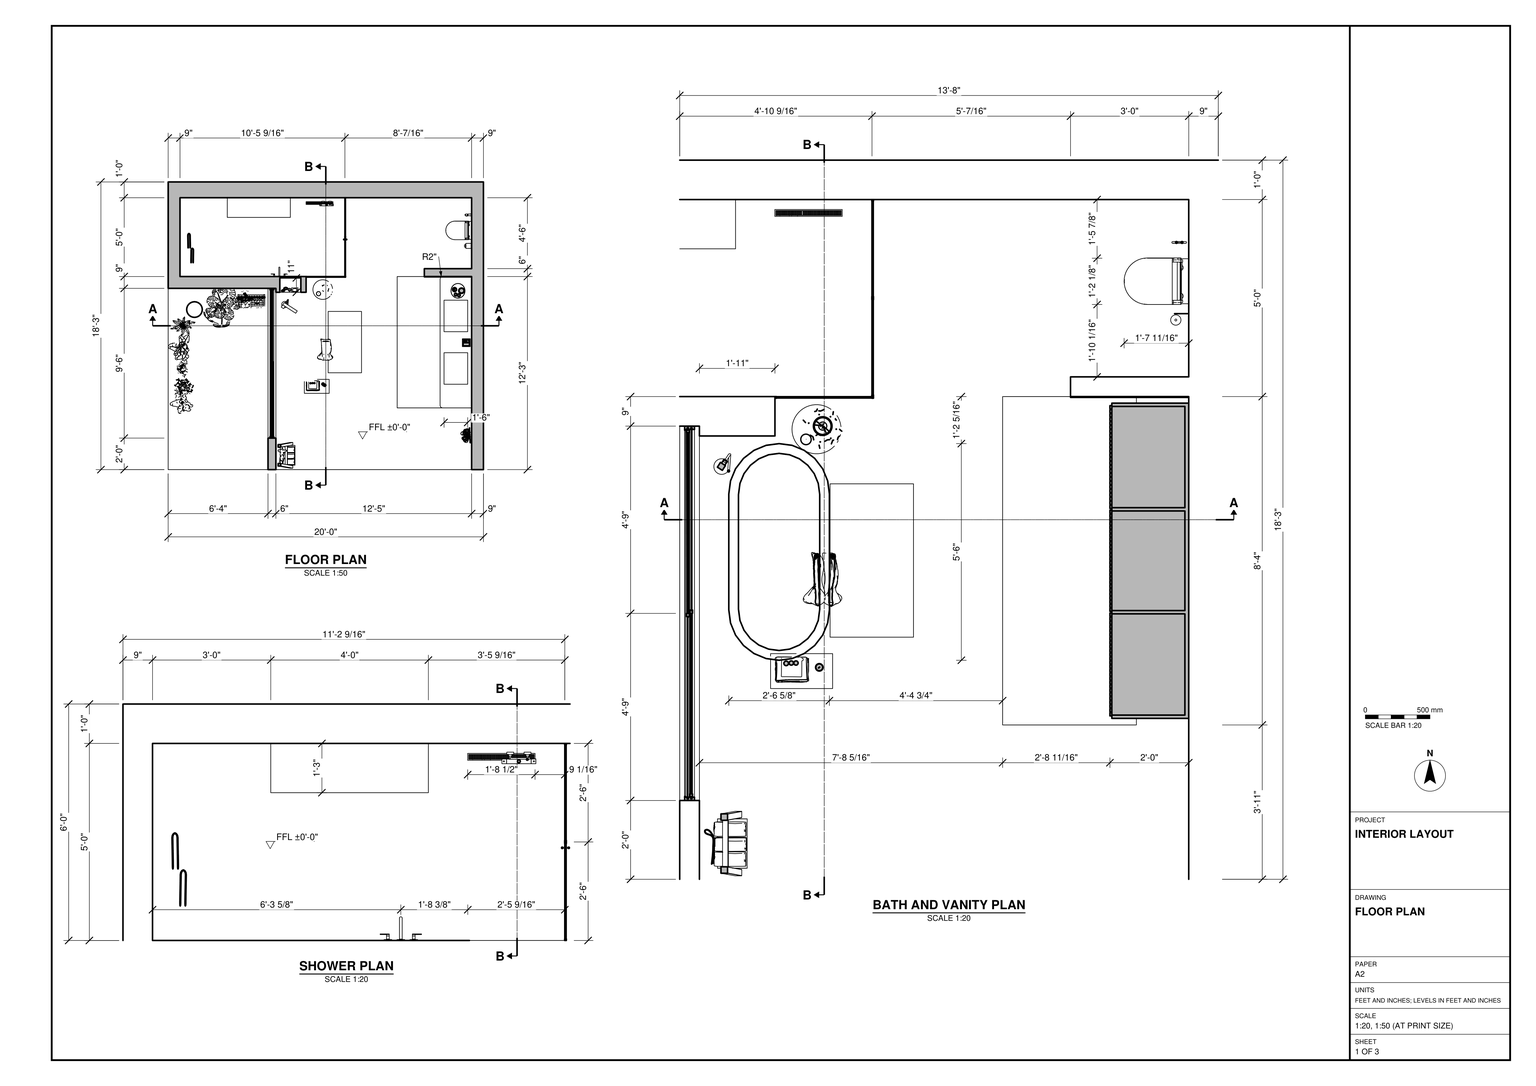
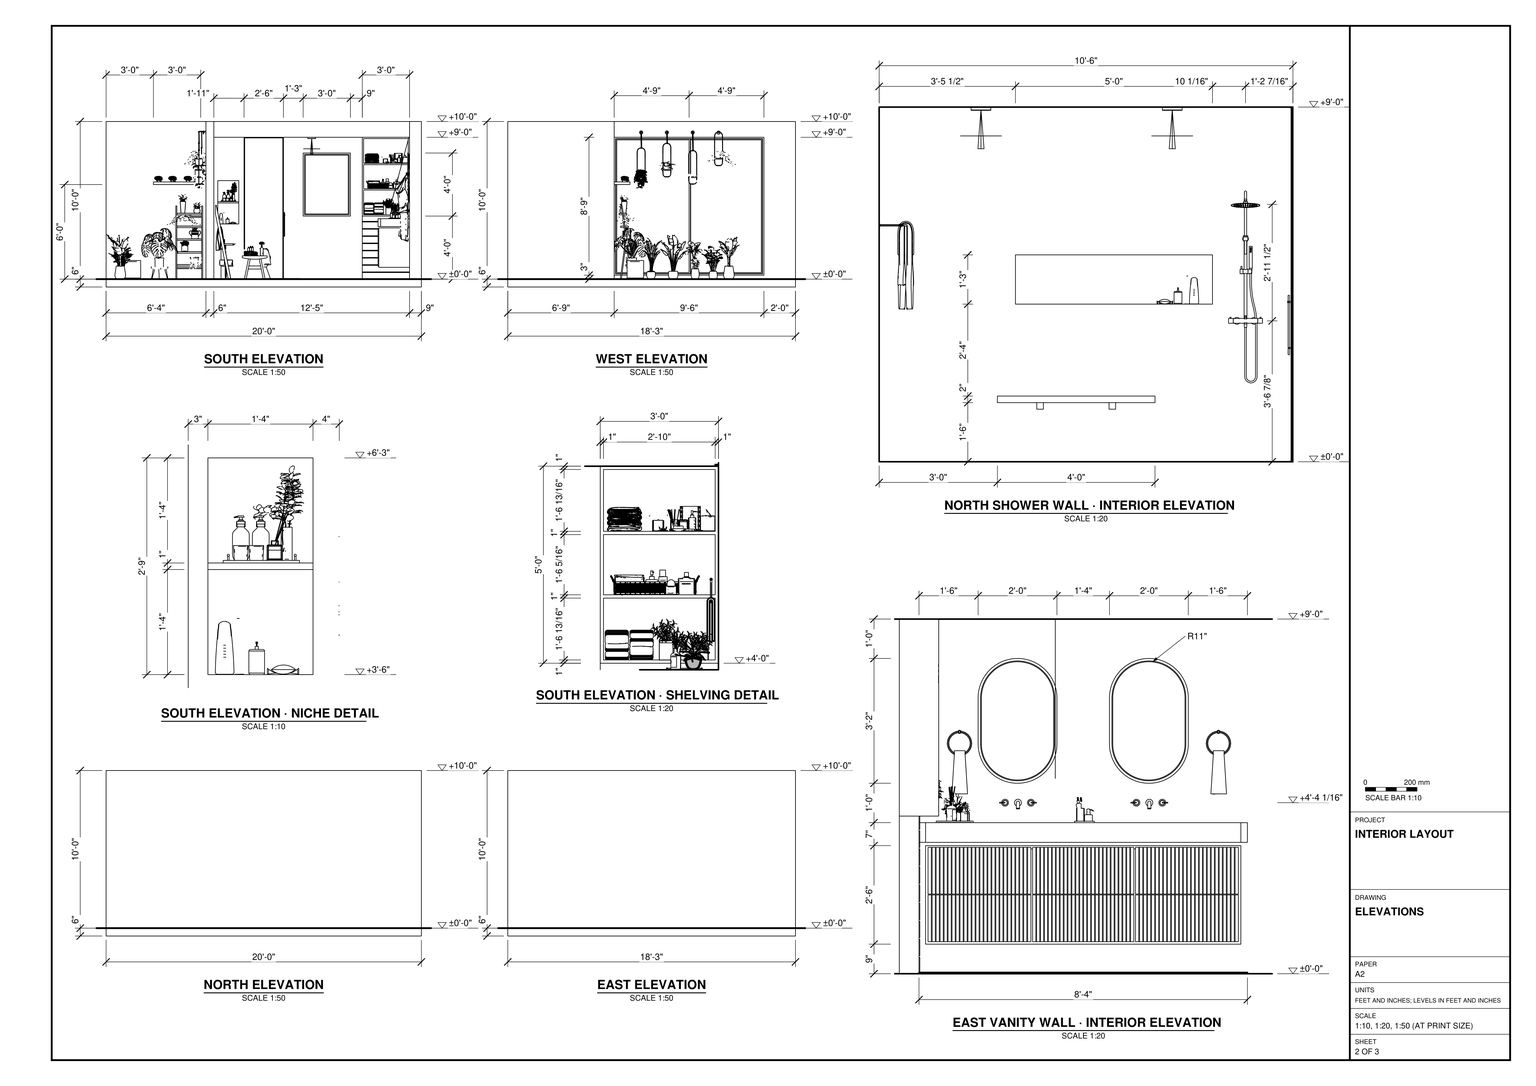
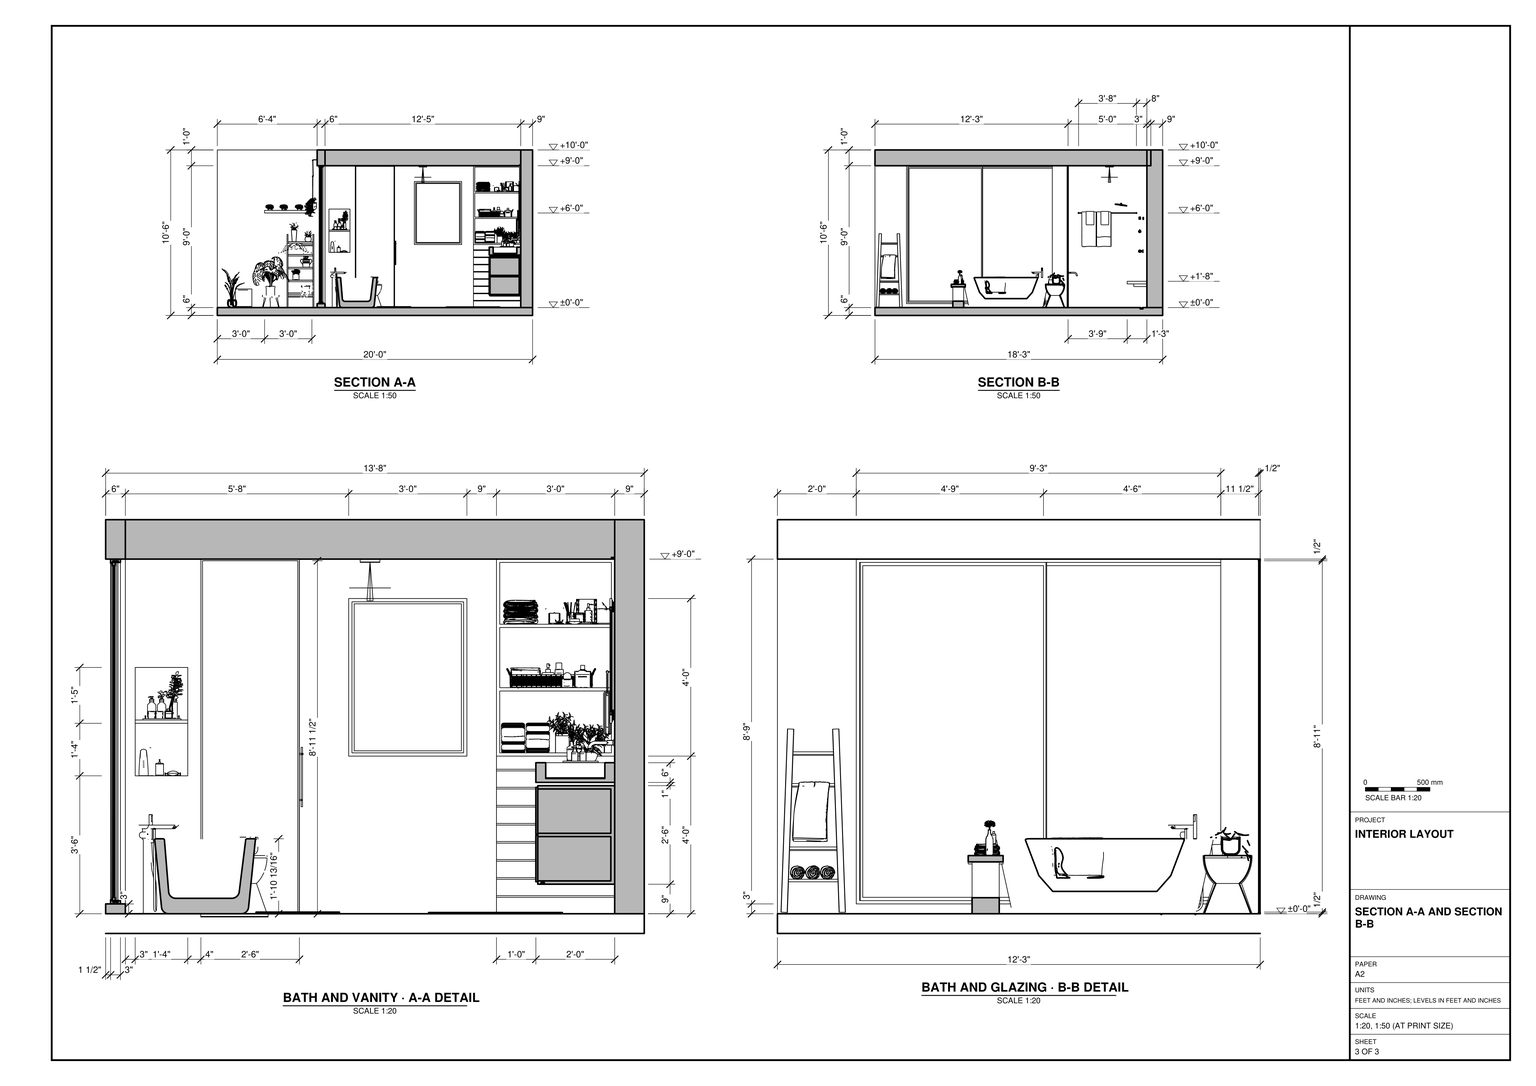
Build the bathroom interior in SketchUp from task_files/diagram_01.pdf. Work in feet and inches. The overall model is 20'-0" wide by 18'-3" deep by 10'-6" high, with the finished floor at ±0'-0". Use the floor plan to locate the walls, partitions and openings, and the sections to set their heights. Model the 6" floor slab and the 1'-0" overhead slab, keeping the planted area outside the enclosed bathroom as shown in section A-A.

Place the shower at the northwest corner and the toilet against the east wall in the northeast recess. Include the shower screen, fittings, wall recess and bench. Set the freestanding tub lengthwise beside the west glazing, facing the double vanity across the room. Use the enlarged plans and elevations to size the tub, the raised vanity cabinet, its countertop and basins, and the mirrors above. Detail the open shelving and the divided wall niche as shown in section A-A. Include the towel stand, bath-side accessories and planting where shown.

Decor and loose items may be any suitable library components. Keep the walls, slabs, roof and each furniture or joinery piece in separate groups or components, and use components for repeated parts. Save one SketchUp model as output_files/bathroom_with_a_freestanding_tub_and_double_vanity.skp.

# SketchUp Ruby script. Lengths in inches.
U = 1.inch
M = Sketchup.active_model
def pt(a) = Geom::Point3d.new(a.map { |v| v * U })
def face(e, loops, mat)
  f = e.add_face(loops[0].map { |a| pt(a) })
  loops[1..].each { |l| e.add_face(l.map { |a| pt(a) }).erase! }
  f.material = f.back_material = mat if mat
  f
end
# faces: each face lists its corners as indices into pts; further lists are holes
def faces(e, pts, list, mat = nil) = list.each { |f| face(e, (f[0].is_a?(Array) ? f : [f]).map { |l| l.map { |i| pts[i] } }, mat) }
# xy, xz, yz: faces in a plane at the given z, y or x. An outline is a flat list of corners, or four numbers for a rectangle; further outlines are holes
def ring(l) = l.size == 4 ? [[l[0], l[1]], [l[2], l[1]], [l[2], l[3]], [l[0], l[3]]] : l.each_slice(2).to_a
def flat(e, list, mat, &to3) = list.each { |f| face(e, (f[0].is_a?(Array) ? f : [f]).map { |l| ring(l).map { |u, v| to3.(u, v) } }, mat) }
def xy(e, z, list, mat = nil) = flat(e, list, mat) { |x, y| [x, y, z] }
def xz(e, y, list, mat = nil) = flat(e, list, mat) { |x, z| [x, y, z] }
def yz(e, x, list, mat = nil) = flat(e, list, mat) { |y, z| [x, y, z] }
def lines(e, pts, list) = list.each { |a, b| e.add_line(pt(pts[a]), pt(pts[b])) }
# prism: a flat outline (further loops are holes) pulled along v
def prism(e, loops, v, mat = nil)
  f = face(e, loops, mat); d = Geom::Vector3d.new(v.map { |x| x * U })
  f.pushpull(f.normal.samedirection?(d) ? d.length : -d.length)
end
def box(e, o, s, mat = nil) = prism(e, [[o, [o[0] + s[0], o[1], o[2]], [o[0] + s[0], o[1] + s[1], o[2]], [o[0], o[1] + s[1], o[2]]]], [0, 0, s[2]], mat)
def at(x, y, z, deg = 0) = Geom::Transformation.translation(pt([x, y, z])) * Geom::Transformation.rotation(ORIGIN, Z_AXIS, deg.degrees)
def axes(o, x, y, z) = Geom::Transformation.new([*x, 0, *y, 0, *z, 0, *pt(o).to_a, 1])
def part(name) = M.definitions.add(name)
# library, detail: a bought-in or finely detailed component or shape, given as its bounding box
def library(name, o, s) = part(name).tap { |d| box(d.entities, o, s) }
def detail(e, o, s) = box(e.add_group.entities, o, s)
def put(e, d, t, mat = nil) = e.add_instance(d, t).tap { |i| i.material = mat if mat }
def group(e, t, mat = nil) = e.add_group.tap { |g| g.transformation = t; g.material = mat if mat }.entities
root = M.entities
M.materials.add("1467 AP 9475 Shining Blue").color = [208, 218, 214]
M.materials.add("BANANA_BIG_STVOL_1").color = [93, 83, 53]
M.materials.add("Goldfish-custom-shape__54193.1487305638").color = [111, 138, 137]
M.materials.add("POT_TEXTURE_1").color = [172, 172, 172]
M.materials.add("POT_TEXTURE_2").color = [160, 154, 144]
M.materials.add("Shelves Light").color = [249, 232, 196]
M.materials.add("Steel_ Copper_ Metal_ Aluminium").color = [30, 30, 30]
M.materials.add("[Carrera Marble]").color = [207, 207, 207]
M.materials.add("[Color A01]").color = [127, 123, 119]
M.materials.add("[Marble Carrara Gold Floor Tile]").color = [221, 221, 221]
M.materials.add("[Metal Seamed]").color = [67, 65, 65]
M.materials.add("[Stone Brushed Khaki]").color = [196, 204, 211]
M.materials.add("[Tile Travertine 2 inch]").color = [56, 54, 50]
M.materials.add("[Wood Floor]").color = [107, 58, 35]
M.materials.add("[Wood Veneer 01]").color = [87, 43, 40]
M.materials.add("[Wood Veneer 01]1").color = [120, 70, 37]
M.materials.add("soil1").color = [68, 55, 47]
M.materials.add("white_concrete_pot1").color = [212, 211, 204]
M.materials.add("wood_1").color = [140, 119, 94]
c1 = library("skp31A6",[-6.04,-1.48,32.125],[7.16,7.43,5.2])
c2 = library("t3",[21.64,8.43,0],[7.57,4.96,6.27])
c3 = library("bathroom accessories",[-9.65,-7.51,0],[20.13,16.97,7.61])
c4 = library("interior plants_leaves_small",[-1.83,-3.05,0],[40.47,20.87,24.79])
c5 = library("Wall hung toilet",[0.42,0,0],[26.94,19.69,42.125])
c6 = library("bain4",[0,0,0],[65.98,62.12,30.23])
c7 = library("Bathroom stool",[0,0,0],[19.9375,11.76,29.04])
c8 = library("JEE-O slimline shower set bronze\#1",[0.04,-0.03,-18.98],[11.61,24.11,65.69])
c9 = part("Goldfish Aqua Runner")
box(c9.entities,[0,0,0],[43.79,100,0.375],"Goldfish-custom-shape__54193.1487305638")
c10 = library("Wall Tap 1",[0,0,0],[12.6,7.22,3.6875])
c11 = library("Hand Towel on Rack",[0,0,0],[3.03,7.5,19.47])
c12 = library("Untitled",[118.83,25.61,-0.38],[19.68,14.54,56.29])
c13 = library("Bathrobe with hooks",[0,0,-0.08],[18.125,10.02,52.34])
c14 = library("Perspective CM",[-13.58,-5.03,0],[27.16,11.23,7.55])
c15 = library("Bathroom accessories \#1",[0,0,0],[11.95,10.24,10.01])
c16 = library("Bahtoorm accessories \#2",[0,1.49,0],[12.27,10,14.78])
c17 = library("Untitled\#1",[35.54,-0.34,0],[6.02,6,7.73])
c18 = library("Bathroom Stool and Styling",[15.82,12.47,0],[25.92,25.93,28.18])
c19 = library("Scara cu plante",[-7.66,-9.41,-0.15],[30.59,22.83,66.38])
c20 = library("plant\#1",[-21.34,-27.21,-0.38],[41.91,41.15,38.97])
c21 = library("Plant\#2",[0,0,0],[12.59,12.59,14.16])
c22 = library("Group\#119",[-312.76,2118.02,370.79],[80.37,61.43,57.53])
c23 = library("Group\#164",[-146.29,2044.53,349.125],[81,53.32,37.9])
c24 = library("Group\#231",[-236.03,2064.57,238.29],[378.97,266.89,1422.96])
c25 = library("Group\#132",[-392.38,2142.99,345.23],[79.77,60.6,39.05])
c26 = library("Group\#193",[-390.04,2074.71,363.78],[77.3,84.83,61.55])
c27 = library("Group\#142",[-389.63,2051.04,359.41],[56.81,81.38,37.86])
c28 = library("Group\#146",[-362.86,1963.26,351.01],[55.56,80.44,37.9])
c29 = library("Group\#163",[-200.52,1998.86,370.22],[77.15,68.38,35.39])
c30 = library("Group\#184",[-480.58,1843.32,11.96],[467.85,466.24,378.92])
c31 = library("Group\#133",[-433.57,2042.61,369.7],[71.79,72.8,37.85])
c32 = library("Group\#130",[-148.5,2084.1,354.63],[73.89,71.73,39.48])
c33 = library("Group\#205",[-372.4375,2154.5,374],[76.125,67.08,39.0625])
c34 = library("Group\#206",[-275.5,2156.34,352.11],[71.39,73.27,44.69])
c35 = library("Group\#174",[-143.56,2061.14,371.42],[79.79,63.19,51.3])
c36 = library("Group\#192",[-363.89,1895.22,354.63],[76.92,66.54,39.48])
c37 = library("Group\#176",[-145.08,2015.32,369.99],[82.29,54.05,37.9])
c38 = library("Group\#203",[-315.77,2202.04,371],[80.74,54.44,37.85])
c39 = library("Group\#194",[-419.21,1941.11,355.02],[73.1,71.21,39.06])
c40 = library("Group\#199",[-229.79,1894.04,351.01],[79.82,63.55,37.9])
c41 = library("Group\#210",[-234.26,2180.97,367.05],[50.63,74.65,43.95])
c42 = library("Group\#213",[-904.81,1865.01,156.3],[624.43,217.34,1227.7])
c43 = library("Group\#214",[-312.51,1611.52,263.78],[120.52,408.52,1275.1])
c44 = library("Group\#217",[-571.16,1736.08,232.33],[294.08,306.57,1438.75])
c45 = library("Group\#222",[-273.21,1593.22,47.51],[374.54,419.07,1416.6])
c46 = library("Group\#123",[-202.35,1900.5,372.29],[58.53,80.11,50.06])
c47 = library("Group\#135",[-432.01,1984.38,372.6875],[64.1,75.95,39.0625])
c48 = library("Group\#168",[-310.7,1952.62,354.63],[79.53,58.52,39.48])
c49 = library("Group\#134",[-374.28,1979.7,369.99],[51.81,82.66,37.9])
c50 = library("Group\#201",[-397.18,1916.74,372.44],[70.02,74.57,49.25])
c51 = library("Group\#208",[-236.3,2186.8,344.47],[79.26,62.91,39.06])
c52 = library("Group\#122",[-161.07,2117.49,373.61],[81.25,53.73,39.48])
c53 = library("Group\#212",[-431.9,1883.46,368.72],[373.65,376.39,18.61])
c54 = library("Group\#167",[-340.96,1970.4,361.28],[81.22,51.59,61.62])
c55 = library("Group\#179",[-272.7,1884.51,369.99],[80.39,55.87,37.9])
c56 = library("Group\#153",[-330.83,2117.69,370.2],[61.83,80.2,35.55])
c57 = library("Group\#209",[-366.3125,2177.8,359.41],[79.9,61.23,37.86])
c58 = library("Group\#145",[-435.875,2067.96,347.82],[58.32,80.53,38.29])
c59 = library("Group\#207",[-183.79,2161.45,371.25],[72.43,70.21,54.35])
c60 = library("Group\#221",[-208.23,2037.18,75.37],[621.09,225.61,1251.82])
c61 = library("Group\#225",[-675.58,1862.05,152.55],[378.81,196.01,1743.84])
c62 = library("Group\#226",[-257.06,2048.08,160.05],[394.6,177.93,1743.83])
c63 = library("Group\#228",[-344.84,1500.61,160.55],[176.35,551.19,1921.45])
c64 = library("Group\#229",[-231.77,1913.24,119.96],[448.93,143.84,1582.05])
c65 = library("Group\#230",[-616.67,2098.6,178.29],[331.19,111.16,1177.92])
c66 = library("Group\#223",[-527.15,2088.47,150.96],[267.01,328.12,1599.25])
c67 = library("Group\#232",[-792.12,2067.32,152.13],[549.56,259.52,1931.8])
c68 = library("Group\#234",[-281.17,2118.67,243.77],[133.23,408.71,1313.3])
c69 = part("Potted houseplant \#1")
g1 = group(c69.entities,at(904.81,-1500.61,-11.96),"white_concrete_pot1")
detail(g1,[-222.14,2117.95,372.07],[61.87,75.41,50.35])
put(c69.entities,c22,at(904.81,-1500.61,-11.96),"white_concrete_pot1")
g2 = group(c69.entities,at(904.81,-1500.61,-11.96),"white_concrete_pot1")
detail(g2,[-313.93,1881.02,351.21],[70.15,73.18,37.2])
g3 = group(c69.entities,at(904.81,-1500.61,-11.96),"white_concrete_pot1")
detail(g3,[-209.1,1970.26,378.89],[50.57,81.04,37.2])
put(c69.entities,c23,at(904.81,-1500.61,-11.96),"white_concrete_pot1")
put(c69.entities,c24,at(904.81,-1500.61,-11.96))
put(c69.entities,c25,at(904.81,-1500.61,-11.96),"white_concrete_pot1")
put(c69.entities,c26,at(904.81,-1500.61,-11.96),"white_concrete_pot1")
put(c69.entities,c27,at(904.81,-1500.61,-11.96),"white_concrete_pot1")
put(c69.entities,c28,at(904.81,-1500.61,-11.96),"white_concrete_pot1")
g4 = group(c69.entities,at(904.81,-1500.61,-11.96),"white_concrete_pot1")
detail(g4,[-129.49,1972.75,359.91],[55.59,80.76,37.2])
put(c69.entities,c29,at(904.81,-1500.61,-11.96),"white_concrete_pot1")
g5 = group(c69.entities,at(904.81,-1500.61,-11.96),"white_concrete_pot1")
detail(g5,[-333.13,1892.25,370.19],[61.39,79.4,37.2])
put(c69.entities,c30,at(904.81,-1500.61,-11.96),"POT_TEXTURE_1")
put(c69.entities,c31,at(904.81,-1500.61,-11.96),"white_concrete_pot1")
put(c69.entities,c32,at(904.81,-1500.61,-11.96),"white_concrete_pot1")
g6 = group(c69.entities,at(904.81,-1500.61,-11.96),"white_concrete_pot1")
detail(g6,[-270.91,2176.57,345.18],[52.11,82.01,38.29])
g7 = group(c69.entities,at(904.81,-1500.61,-11.96),"white_concrete_pot1")
detail(g7,[-195.71,2019.1875,371.11],[58.98,81.18,37.2])
g8 = group(c69.entities,at(904.81,-1500.61,-11.96),"white_concrete_pot1")
detail(g8,[-319.36,2078.81,339.18],[76.07,69.08,39.48])
put(c69.entities,c33,at(904.81,-1500.61,-11.96),"white_concrete_pot1")
put(c69.entities,c34,at(904.81,-1500.61,-11.96),"white_concrete_pot1")
g9 = group(c69.entities,at(904.81,-1500.61,-11.96),"white_concrete_pot1")
detail(g9,[-417.64,2112.53,369.82],[65.44,79.59,38.29])
put(c69.entities,c35,at(904.81,-1500.61,-11.96),"white_concrete_pot1")
put(c69.entities,c36,at(904.81,-1500.61,-11.96),"white_concrete_pot1")
put(c69.entities,c37,at(904.81,-1500.61,-11.96),"white_concrete_pot1")
g10 = group(c69.entities,at(904.81,-1500.61,-11.96),"white_concrete_pot1")
detail(g10,[-240.6,2054.85,378.89],[71.5,72.03,37.2])
put(c69.entities,c38,at(904.81,-1500.61,-11.96),"white_concrete_pot1")
put(c69.entities,c39,at(904.81,-1500.61,-11.96),"white_concrete_pot1")
put(c69.entities,c40,at(904.81,-1500.61,-11.96),"white_concrete_pot1")
g11 = group(c69.entities,at(904.81,-1500.61,-11.96),"white_concrete_pot1")
detail(g11,[-249.82,2117.53,359.91],[58.07,81.25,37.2])
put(c69.entities,c41,at(904.81,-1500.61,-11.96),"white_concrete_pot1")
put(c69.entities,c42,at(904.81,-1500.61,-11.96))
put(c69.entities,c43,at(904.81,-1500.61,-11.96))
put(c69.entities,c44,at(904.81,-1500.61,-11.96))
put(c69.entities,c45,at(904.81,-1500.61,-11.96))
g12 = group(c69.entities,at(904.81,-1500.61,-11.96),"white_concrete_pot1")
detail(g12,[-435.4375,2027.54,350.71],[78.74,62.6,37.86])
put(c69.entities,c46,at(904.81,-1500.61,-11.96),"white_concrete_pot1")
g13 = group(c69.entities,at(904.81,-1500.61,-11.96),"white_concrete_pot1")
detail(g13,[-173.8,2126.25,354.63],[80.17,60.53,39.48])
g14 = group(c69.entities,at(904.81,-1500.61,-11.96),"white_concrete_pot1")
detail(g14,[-222.96,2066.75,359.91],[63.77,78.21,37.2])
put(c69.entities,c47,at(904.81,-1500.61,-11.96),"white_concrete_pot1")
g15 = group(c69.entities,at(904.81,-1500.61,-11.96),"white_concrete_pot1")
detail(g15,[-183.125,1913.38,330.04],[66.78,77.69,39.48])
put(c69.entities,c48,at(904.81,-1500.61,-11.96),"white_concrete_pot1")
g16 = group(c69.entities,at(904.81,-1500.61,-11.96),"white_concrete_pot1")
detail(g16,[-152,1936.85,378.89],[64.46,79.76,37.2])
g17 = group(c69.entities,at(904.81,-1500.61,-11.96),"white_concrete_pot1")
detail(g17,[-284.65,1933.22,373.64],[80.83,55.23,37.2])
put(c69.entities,c49,at(904.81,-1500.61,-11.96),"white_concrete_pot1")
g18 = group(c69.entities,at(904.81,-1500.61,-11.96),"white_concrete_pot1")
detail(g18,[-263.49,1923.54,359.91],[75.98,66.75,37.2])
put(c69.entities,c50,at(904.81,-1500.61,-11.96),"white_concrete_pot1")
g19 = group(c69.entities,at(904.81,-1500.61,-11.96),"white_concrete_pot1")
detail(g19,[-167.97,1940.97,354.63],[66.78,77.7,39.48])
put(c69.entities,c51,at(904.81,-1500.61,-11.96),"white_concrete_pot1")
g20 = group(c69.entities,at(904.81,-1500.61,-11.96),"white_concrete_pot1")
detail(g20,[-214.75,1956.59,330.04],[66.78,77.69,39.48])
put(c69.entities,c52,at(904.81,-1500.61,-11.96),"white_concrete_pot1")
put(c69.entities,c53,at(904.81,-1500.61,-11.96),"white_concrete_pot1")
put(c69.entities,c54,at(904.81,-1500.61,-11.96),"white_concrete_pot1")
g21 = group(c69.entities,at(904.81,-1500.61,-11.96),"white_concrete_pot1")
detail(g21,[-282.5625,1934.21,389.56],[81.1,59.19,35.03])
put(c69.entities,c55,at(904.81,-1500.61,-11.96),"white_concrete_pot1")
g22 = group(c69.entities,at(904.81,-1500.61,-11.96),"white_concrete_pot1")
detail(g22,[-394.5,2036.48,359.91],[79.58,64.84,37.2])
put(c69.entities,c56,at(904.81,-1500.61,-11.96),"white_concrete_pot1")
put(c69.entities,c57,at(904.81,-1500.61,-11.96),"white_concrete_pot1")
put(c69.entities,c58,at(904.81,-1500.61,-11.96),"white_concrete_pot1")
put(c69.entities,c59,at(904.81,-1500.61,-11.96),"white_concrete_pot1")
put(c69.entities,c60,at(904.81,-1500.61,-11.96))
put(c69.entities,c61,at(904.81,-1500.61,-11.96))
put(c69.entities,c62,at(904.81,-1500.61,-11.96))
put(c69.entities,c63,at(904.81,-1500.61,-11.96))
put(c69.entities,c64,at(904.81,-1500.61,-11.96))
put(c69.entities,c65,at(904.81,-1500.61,-11.96))
put(c69.entities,c66,at(904.81,-1500.61,-11.96))
put(c69.entities,c67,at(904.81,-1500.61,-11.96))
put(c69.entities,c68,at(904.81,-1500.61,-11.96))
c70 = library("Group\#242",[-662.41,217.3,320.04],[397.32,658.3,1732.06])
c71 = library("Group\#244",[-299.2,181.55,262.58],[360.65,735.71,1258.34])
c72 = library("Group\#239",[-1038.76,656.55,345.34],[733.18,460.51,2065.7])
c73 = library("Group\#237",[-445.29,890.31,329.28],[284.3,304.08,2023.29])
c74 = library("Group\#240",[-733.48,439.625,202.64],[456.28,533.12,1536.78])
c75 = library("Group\#243",[-455.56,899.32,410.78],[341.21,610.33,1581.5])
c76 = library("Group\#236",[-516.34,626.77,-4.5625],[517.73,515.95,418.98])
c77 = library("Group\#241",[-249.24,914.85,310.18],[345.55,647.95,1307.93])
c78 = library("Group\#238",[-277.97,488.68,287.26],[362.84,405.94,1768.54])
c79 = library("Group\#235",[-468.76,669.89,380.1875],[424.36,427.47,41.99])
c80 = part("Potted tropical plant")
put(c80.entities,c70,at(1038.76,-181.55,4.5625))
put(c80.entities,c71,at(1038.76,-181.55,4.5625))
put(c80.entities,c72,at(1038.76,-181.55,4.5625))
put(c80.entities,c73,at(1038.76,-181.55,4.5625))
put(c80.entities,c74,at(1038.76,-181.55,4.5625))
put(c80.entities,c75,at(1038.76,-181.55,4.5625))
put(c80.entities,c76,at(1038.76,-181.55,4.5625),"POT_TEXTURE_1")
put(c80.entities,c77,at(1038.76,-181.55,4.5625))
put(c80.entities,c78,at(1038.76,-181.55,4.5625))
put(c80.entities,c79,at(1038.76,-181.55,4.5625),"soil1")
c81 = library("Group\#248",[-246.45,-349.05,558.47],[136.91,100.49,66.1])
c82 = library("Group\#251",[-264.68,-415.73,1484.11],[304.64,209.69,227.41])
c83 = library("Group\#259",[-357.04,-394.18,1447.05],[213.62,306.36,356.95])
c84 = library("Group\#246",[-447.02,-464.95,536.35],[343.73,346.24,39.39])
c85 = library("Group\#247",[-394.9,-448.99,911.74],[90.19,96.88,85.93])
c86 = library("Group\#258",[-424,-312.27,817.53],[158.81,108.06,136.45])
c87 = library("Group\#262",[-409.02,-515.05,915.53],[69.62,77.27,65.47])
c88 = library("Group\#266",[-548.25,-262.82,1459.54],[373.26,352.35,568])
c89 = library("Group\#274",[-492.14,-508.4,-4.15],[433.72,431.71,567.03])
c90 = library("Group\#269",[-293.78,-482.77,597.9],[158.75,112.78,159.87])
c91 = library("Group\#252",[-545.09,-386.51,922.3125],[300.25,219.65,227.33])
c92 = library("Group\#271",[-292.81,-667.38,1418.14],[215.17,356.07,188.87])
c93 = library("Group\#254",[-292.14,-288.9,1281.79],[169.55,204.34,203.36])
c94 = library("Group\#260",[-568.91,-444.37,1285.4],[307.6,179.39,277.93])
c95 = library("Group\#257",[-341.93,-403.49,744.8125],[64.83,96.32,132.15])
c96 = library("Group\#245",[-258.04,-282.68,604.05],[115.53,137.01,52.63])
c97 = library("Group\#253",[-304.79,-269.16,622.65],[82.06,111.89,102.57])
c98 = library("Group\#261",[-388.93,-514.39,838.93],[89.79,77.73,82.08])
c99 = library("Group\#263",[-295.03,-516.52,742.34],[68.71,141.75,78.67])
c100 = library("Group\#270",[-422.77,-235.4,843.61],[178.54,197.77,233.54])
c101 = library("Group\#264",[-498.98,-524.4,908.45],[120.83,107.95,112.98])
c102 = library("Group\#267",[-321.08,-139.66,1308.49],[285.55,393.29,221.53])
c103 = library("Group\#265",[-278.4,-571.99,1530.91],[311.57,345.77,423.62])
c104 = library("Group\#268",[-387.74,-136.11,1470.07],[230,321.58,230.27])
c105 = library("Group\#256",[-244.55,-305.59,1009.46],[103.13,76.81,77.34])
c106 = library("Group\#273",[-385.21,-446.52,494.02],[160.93,321.12,1142.36])
c107 = library("Group\#249",[-249.18,-250.59,980.93],[152.21,116.16,134.05])
c108 = library("Group\#250",[-438.92,-265.61,702.3],[171.52,146.16,133.5])
c109 = part("Potted houseplant")
p = [[568.91,667.38,4.15],[569.91,667.38,4.15],[569.91,668.38,4.15]]
lines(c109.entities,p,[[0,1],[1,2],[2,0]])
put(c109.entities,c81,at(568.91,667.38,4.15))
put(c109.entities,c82,at(568.91,667.38,4.15))
put(c109.entities,c83,at(568.91,667.38,4.15))
put(c109.entities,c84,at(568.91,667.38,4.15),"soil1")
put(c109.entities,c85,at(568.91,667.38,4.15))
put(c109.entities,c86,at(568.91,667.38,4.15))
put(c109.entities,c87,at(568.91,667.38,4.15))
put(c109.entities,c88,at(568.91,667.38,4.15))
put(c109.entities,c89,at(568.91,667.38,4.15),"POT_TEXTURE_2")
put(c109.entities,c90,at(568.91,667.38,4.15))
put(c109.entities,c91,at(568.91,667.38,4.15))
put(c109.entities,c92,at(568.91,667.38,4.15))
put(c109.entities,c93,at(568.91,667.38,4.15))
put(c109.entities,c94,at(568.91,667.38,4.15))
put(c109.entities,c95,at(568.91,667.38,4.15))
put(c109.entities,c96,at(568.91,667.38,4.15))
put(c109.entities,c97,at(568.91,667.38,4.15))
put(c109.entities,c98,at(568.91,667.38,4.15))
put(c109.entities,c99,at(568.91,667.38,4.15))
put(c109.entities,c100,at(568.91,667.38,4.15))
put(c109.entities,c101,at(568.91,667.38,4.15))
put(c109.entities,c102,at(568.91,667.38,4.15))
put(c109.entities,c103,at(568.91,667.38,4.15))
put(c109.entities,c104,at(568.91,667.38,4.15))
put(c109.entities,c105,at(568.91,667.38,4.15))
put(c109.entities,c106,at(568.91,667.38,4.15),"wood_1")
put(c109.entities,c107,at(568.91,667.38,4.15))
put(c109.entities,c108,at(568.91,667.38,4.15))
c110 = library("Group\#283",[-640.625,-1318.37,287.11],[396.64,314.81,689.96])
c111 = library("Group\#277",[-513.94,-1201.2,195.17],[480.66,557.42,1160.08])
c112 = library("Group\#279",[-208.03,-1336.63,286.21],[381.72,484.79,1145.39])
c113 = library("Group\#286",[-619.83,-1636.3,288.9],[316.15,456.61,1171.28])
c114 = library("Group\#287",[-738.91,-1210.08,301],[426.4,388.88,1000.79])
c115 = library("Group\#289",[-208.33,-1511.76,297.04],[508.2,421.96,1258.76])
c116 = library("Group\#278",[-545.36,-1775.03,287.125],[412.21,432,920.68])
c117 = library("Group\#284",[-750.24,-1478.51,301.56],[423.84,451.05,998.69])
c118 = library("Group\#282",[-245.33,-1174.2,301.22],[356.02,306.31,608.34])
c119 = library("Group\#276",[-487.23,-1483.58,-4.71],[450.86,446.99,418.38])
c120 = library("Group\#291",[-445.7,-1606.55,154.18],[255.44,283.57,849.28])
c121 = library("Group\#292",[-390.1,-1177.12,195.59],[220.93,265.44,790.12])
c122 = library("Group\#294",[-480.32,-1333.42,295.8],[424.49,356.06,1482.77])
c123 = library("Group\#295",[-378.01,-1245.98,305.66],[422.15,474.55,1267.42])
c124 = library("Group\#281",[-163.65,-1622.09,292.29],[406.18,374.8,780.12])
c125 = library("Group\#290",[-384.8,-1640.99,300.61],[422.68,348.03,1297.96])
c126 = library("Group\#275",[-429.18,-1441.17,362.05],[345.84,348.28,45.35])
c127 = library("Group\#293",[-208.0625,-1498.77,286.27],[547.26,435.76,1075.6])
c128 = library("Group\#288",[-172.82,-1329.68,294.68],[502.85,397.72,955.79])
c129 = library("Group\#285",[-426.76,-1753.59,287.48],[479.67,412.35,1049.19])
c130 = part("Potted palm")
put(c130.entities,c110,at(750.24,1775.03,4.71))
put(c130.entities,c111,at(750.24,1775.03,4.71))
put(c130.entities,c112,at(750.24,1775.03,4.71))
put(c130.entities,c113,at(750.24,1775.03,4.71))
put(c130.entities,c114,at(750.24,1775.03,4.71))
put(c130.entities,c115,at(750.24,1775.03,4.71))
put(c130.entities,c116,at(750.24,1775.03,4.71))
put(c130.entities,c117,at(750.24,1775.03,4.71))
put(c130.entities,c118,at(750.24,1775.03,4.71))
put(c130.entities,c119,at(750.24,1775.03,4.71),"POT_TEXTURE_1")
put(c130.entities,c120,at(750.24,1775.03,4.71))
put(c130.entities,c121,at(750.24,1775.03,4.71))
put(c130.entities,c122,at(750.24,1775.03,4.71))
put(c130.entities,c123,at(750.24,1775.03,4.71))
put(c130.entities,c124,at(750.24,1775.03,4.71))
put(c130.entities,c125,at(750.24,1775.03,4.71))
put(c130.entities,c126,at(750.24,1775.03,4.71),"soil1")
put(c130.entities,c127,at(750.24,1775.03,4.71))
put(c130.entities,c128,at(750.24,1775.03,4.71))
put(c130.entities,c129,at(750.24,1775.03,4.71))
c131 = library("Group\#296",[-480.3,-2300.47,677.45],[398.14,398.43,28.25])
c132 = library("Group\#297",[-336.38,-2175.79,614.41],[133.99,147.1,560.64])
c133 = library("Group\#298",[-311.45,-2362.85,663.67],[597.01,322.07,1007.38])
c134 = library("Group\#299",[-330.26,-2159.14,612.04],[116.66,119.22,673.97])
c135 = library("Group\#302",[-667.53,-2111.4375,1071.74],[420.02,555.28,968.03])
c136 = library("Group\#303",[-328.97,-2115.58,1156.29],[117.86,119.42,695.38])
c137 = library("Group\#305",[-943.22,-2312.1875,967.59],[670.63,402.45,1245.73])
c138 = library("Group\#308",[-343.93,-2076.42,1024.91],[285.05,475.82,708.21])
c139 = library("Group\#306",[-568.09,-2386.9,-3.76],[573.62,569.18,700.28])
c140 = library("Group\#309",[-550.09,-2664.39,1031.96],[371.42,533.86,798])
c141 = library("Group\#310",[-308.37,-2556.11,869.35],[483.58,483.6,1385.8])
c142 = part("Potted tropical plant \#1")
put(c142.entities,c131,at(943.22,2664.39,3.76),"soil1")
put(c142.entities,c132,at(943.22,2664.39,3.76),"BANANA_BIG_STVOL_1")
put(c142.entities,c133,at(943.22,2664.39,3.76))
put(c142.entities,c134,at(943.22,2664.39,3.76),"BANANA_BIG_STVOL_1")
put(c142.entities,c135,at(943.22,2664.39,3.76))
put(c142.entities,c136,at(943.22,2664.39,3.76))
put(c142.entities,c137,at(943.22,2664.39,3.76))
put(c142.entities,c138,at(943.22,2664.39,3.76))
put(c142.entities,c139,at(943.22,2664.39,3.76),"POT_TEXTURE_2")
put(c142.entities,c140,at(943.22,2664.39,3.76))
put(c142.entities,c141,at(943.22,2664.39,3.76))
c143 = part("plants\#1")
put(c143.entities,c69,at(-904.81,1500.61,11.96))
put(c143.entities,c80,at(-1038.76,181.55,-4.5625))
put(c143.entities,c109,at(-568.91,-667.38,-4.15))
put(c143.entities,c130,at(-750.24,-1775.03,-4.71))
put(c143.entities,c142,at(-943.22,-2664.39,-3.76))
c144 = library("Umbra+Bolo",[-7.04,-1.89,-4.93],[32.14,86.7,48.29])
c145 = part("Group\#30")
box(c145.entities,[0,0,-0.5],[34,1,0.5])
c146 = library("Group\#5",[-20.5,-2,0],[20.5,100,87])
c147 = library("Group\#14",[0,0,0],[31.13,60.5,108])
c148 = library("Group\#15",[-0.5,0,0],[3,114,105])
c149 = part("wall art6")
g23 = group(c149.entities,at(66.77,0,0.01))
xy(g23,0,[[0,-0.79,39.37,0]],"Steel_ Copper_ Metal_ Aluminium")
xy(g23,0.79,[[0.79,-0.79,38.58,-0.39],[0.79,-0.39,38.58,0]],"Steel_ Copper_ Metal_ Aluminium")
xy(g23,58.27,[[0.79,-0.79,38.58,-0.39],[0.79,-0.39,38.58,0]],"Steel_ Copper_ Metal_ Aluminium")
xy(g23,59.06,[[0,-0.79,39.37,0]],"Steel_ Copper_ Metal_ Aluminium")
xz(g23,-0.79,[[[0,0,39.37,59.06],[0.79,0.79,38.58,58.27]]],"Steel_ Copper_ Metal_ Aluminium")
xz(g23,-0.39,[[0.79,0.79,38.58,58.27]],"[Color A01]")
xz(g23,0,[[[0,0,39.37,59.06],[0.79,0.79,38.58,58.27]],[0.79,0.79,38.58,58.27]],"Steel_ Copper_ Metal_ Aluminium")
yz(g23,0,[[-0.79,0,0,59.06]],"Steel_ Copper_ Metal_ Aluminium")
yz(g23,0.79,[[-0.79,0.79,-0.39,58.27],[-0.39,0.79,0,58.27]],"Steel_ Copper_ Metal_ Aluminium")
yz(g23,38.58,[[-0.79,0.79,-0.39,58.27],[-0.39,0.79,0,58.27]],"Steel_ Copper_ Metal_ Aluminium")
yz(g23,39.37,[[-0.79,0,0,59.06]],"Steel_ Copper_ Metal_ Aluminium")
c150 = part("Group228\#1")
box(c150.entities,[-18,-24,0],[36,5,0.25])
c151 = part("Group229\#1")
box(c151.entities,[-18,-18.5,0],[36,5,0.25])
c152 = part("Group230\#1")
box(c152.entities,[-18,-13,0],[36,5,0.25])
c153 = part("Group231\#1")
box(c153.entities,[-18,-7.5,0],[36,5,0.25])
c154 = part("Group232\#1")
box(c154.entities,[-18,-2,0],[36,5,0.25])
c155 = part("Group233\#1")
box(c155.entities,[-18,3.5,0],[36,5,0.25])
c156 = part("Group234\#1")
box(c156.entities,[-18,9,0],[36,5,0.25])
c157 = part("Group235\#1")
box(c157.entities,[-18,14.5,0],[36,5,0.25])
c158 = part("Group236\#1")
box(c158.entities,[-18,20,0],[36,4,0.25])
c159 = part("Group226\#1")
put(c159.entities,c150,at(0,0,0))
put(c159.entities,c151,at(0,0,0))
put(c159.entities,c152,at(0,0,0))
put(c159.entities,c153,at(0,0,0))
put(c159.entities,c154,at(0,0,0))
put(c159.entities,c155,at(0,0,0))
put(c159.entities,c156,at(0,0,0))
put(c159.entities,c157,at(0,0,0))
put(c159.entities,c158,at(0,0,0))
c160 = library("Group\#36",[0,0,-25.17],[10.55,45,26.91])
c161 = library("Group\#311",[0,0,0],[36,6.43,12])
c162 = library("Сауна. Дренаж",[0,0,0],[36,3.67,1.375])
c163 = library("Group\#23",[9,0,-60.67],[222,210,60.67])
c164 = library("Group\#52",[0,-0.31,0],[12.93,3.92,8.58])
put(root,c1,axes([199.23,142.59,42.87],[0,-1.41,0],[1.41,0,0],[0,0,1.41]))
put(root,c2,axes([184.26,183.36,49],[0,-1.45,0],[1.45,0,0],[0,0,1.45]))
put(root,c2,axes([191.76,183.36,58.09],[0,-1.45,0],[1.45,0,0],[0,0,-1.45]))
g24 = group(root,at(48,0,0))
put(g24,c3,axes([171.52,145.87,88.17],[1,0,0],[0,0.64822,0],[0,0,1]))
put(g24,c4,axes([162.4,139.53,48.95],[0.54,0,0],[0,0.54,0],[0,0,0.54]))
g25 = group(g24,at(0,0,0),"1467 AP 9475 Shining Blue")
xy(g25,0,[[28,0,28,138,-48,138,-48,219,192,219,192,0,183,0,183,147,147,147,147,153,183,153,183,207,-39,207,-39,147,57,147,57,135,34,135,34,0]])
xy(g25,3,[[28,24,34,138]])
xy(g25,42,[[37,135,53,146]],"[Carrera Marble]")
xy(g25,48,[[147,147,183,153]])
xy(g25,48,[[2.5,207,62.5,213]],"[Carrera Marble]")
xy(g25,58,[[37,145,53,146]])
xy(g25,58,[[37,136,53,144]],"[Carrera Marble]")
xy(g25,58.5,[[37,144,53,145]])
xy(g25,59,[[37,136,53,146]],"[Carrera Marble]")
xy(g25,63,[[2.5,207,62.5,211],[2.5,212,62.5,213]])
xy(g25,63.5,[[2.5,211,62.5,212]])
xy(g25,75,[[37,135,53,144],[37,145,53,146]])
xy(g25,75.5,[[37,144,53,145]])
xy(g25,108,[[28,24,34,138],[34,135,57,147]])
xy(g25,120,[[28,0,34,0,34,147,-39,147,-39,207,183,207,183,0,192,0,192,219,-48,219,-48,138,28,138]])
xz(g25,0,[[28,0,34,120],[183,0,192,120]])
xz(g25,24,[[28,3,34,108]])
xz(g25,135,[[[34,0,57,108],[37,42,53,75]]],"[Stone Brushed Khaki]")
xz(g25,136,[[37,58,53,59]],"[Carrera Marble]")
xz(g25,138,[[-48,0,28,0,28,3,34,3,34,108,28,108,28,120,-48,120]],"1467 AP 9475 Shining Blue")
xz(g25,144,[[37,58,53,58.5],[37,75,53,75.5]])
xz(g25,145,[[37,58,53,58.5],[37,75,53,75.5]])
xz(g25,146,[[37,42,53,58],[37,59,53,75]],"[Carrera Marble]")
xz(g25,147,[[-39,0,-39,120,34,120,34,108,57,108,57,0],[147,0,183,48]])
xz(g25,153,[[147,0,183,48]])
xz(g25,207,[[[-39,0,183,120],[2.5,48,62.5,63]]],"[Stone Brushed Khaki]")
xz(g25,211,[[2.5,63,62.5,63.5]])
xz(g25,212,[[2.5,63,62.5,63.5]])
xz(g25,213,[[2.5,48,62.5,63]],"[Carrera Marble]")
xz(g25,219,[[-48,0,192,120]])
yz(g25,-48,[[138,0,219,120]])
yz(g25,-39,[[147,0,207,120]])
yz(g25,2.5,[[207,48,213,48,213,63,212,63,212,63.5,211,63.5,211,63,207,63]])
yz(g25,28,[[0,0,0,120,138,120,138,108,24,108,24,3,138,3,138,0]],"1467 AP 9475 Shining Blue")
yz(g25,34,[[135,3,138,108]])
yz(g25,34,[[0,0,135,0,135,3,24,3,24,108,147,108,147,120,0,120]],"1467 AP 9475 Shining Blue")
yz(g25,37,[[135,42,146,42,146,58,145,58,145,58.5,144,58.5,144,58,136,58,136,59,146,59,146,75,145,75,145,75.5,144,75.5,144,75,135,75]],"[Carrera Marble]")
yz(g25,53,[[135,42,135,75,144,75,144,75.5,145,75.5,145,75,146,75,146,59,136,59,136,58,144,58,144,58.5,145,58.5,145,58,146,58,146,42]],"[Carrera Marble]")
yz(g25,57,[[135,0,147,108]],"[Stone Brushed Khaki]")
yz(g25,62.5,[[207,48,207,63,211,63,211,63.5,212,63.5,212,63,213,63,213,48]],"[Carrera Marble]")
yz(g25,147,[[147,0,153,48]])
yz(g25,183,[[0,0,0,120,207,120,207,0,153,0,153,48,147,48,147,0]],"1467 AP 9475 Shining Blue")
yz(g25,192,[[0,0,219,120]])
put(g25,c5,at(183,167.95,0,90))
put(g25,c6,axes([99.1875,132.68,0],[0,-1,0],[-1,0,0],[0,0,1]))
put(g25,c7,at(55.66,58.09,0))
put(g25,c8,axes([67.35,182.92,40.89],[0.89,0,0],[0,0.89,0],[0,0,0.89]))
put(g25,c9,axes([126.33,47,0],[0.93,0,0],[0,1,0],[0,0,1]))
put(g25,c10,axes([30.31,154.22,24],[1,0,0],[0,-1,0],[0,0,1]))
put(g25,c11,at(179.6,52.06,54.6875))
put(g25,c11,at(179.6,130.92,54.6875))
put(g25,c12,axes([74.15,139.56,0.38],[0,-1,0],[-1,0,0],[0,0,1]))
put(g25,c13,at(183,17.85,28.74,92.5))
put(g25,c14,at(163.66,146.03,68.83))
put(g25,c15,axes([180.39,130.5,46],[-1.1,0,0],[0,1.1,0],[0,0,1.1]))
put(g25,c16,at(39.32,135.26,59))
put(g25,c17,at(140.39,93.97,46))
put(g25,c18,at(42.98,111.53,0))
put(g25,c19,at(5.07,124.5625,0.15))
put(g25,c20,at(-0.84,127.24,0,-60))
put(g25,c21,at(-34.28,115.57,0))
put(g25,c143,axes([-33.26,80.52,0.07],[0.01419,0,0],[0,0.01419,0],[0,0,0.01419]))
put(g25,c144,at(27.95,122.6,69.5625,180))
g26 = group(g25,at(183,141,48),"[Wood Veneer 01]1")
xy(g26,0,[[-36,0,0,6],[-36,6,0,12]])
xy(g26,1,[[-35,0,-1,11]])
xy(g26,19.83,[[-35,0,-1,9],[-35,10,-1,11]])
xy(g26,20.33,[[-35,9,-1,10]])
xy(g26,20.83,[[-35,0,-1,11]])
xy(g26,39.17,[[-35,0,-1,9],[-35,10,-1,11]])
xy(g26,39.67,[[-35,9,-1,10]])
xy(g26,40.17,[[-35,0,-1,11]])
xy(g26,59,[[-35,0,-1,9],[-35,10,-1,11]])
xy(g26,59.5,[[-35,9,-1,10]])
xy(g26,60,[[-36,0,0,12]])
xz(g26,0,[[[-36,0,0,60],[-35,40.17,-1,59],[-35,1,-1,19.83],[-35,20.83,-1,39.17]]])
xz(g26,9,[[-35,19.83,-1,20.33],[-35,39.17,-1,39.67],[-35,59,-1,59.5]])
xz(g26,10,[[-35,19.83,-1,20.33],[-35,39.17,-1,39.67],[-35,59,-1,59.5]])
xz(g26,11,[[-35,1,-1,19.83],[-35,20.83,-1,39.17],[-35,40.17,-1,59]])
xz(g26,12,[[-36,0,0,60]])
yz(g26,-36,[[0,0,12,60]])
yz(g26,-35,[[0,1,11,1,11,19.83,10,19.83,10,20.33,9,20.33,9,19.83,0,19.83],[0,20.83,11,20.83,11,39.17,10,39.17,10,39.67,9,39.67,9,39.17,0,39.17],[0,40.17,11,40.17,11,59,10,59,10,59.5,9,59.5,9,59,0,59]])
yz(g26,-1,[[0,1,0,19.83,9,19.83,9,20.33,10,20.33,10,19.83,11,19.83,11,1],[0,20.83,0,39.17,9,39.17,9,39.67,10,39.67,10,39.17,11,39.17,11,20.83],[0,40.17,0,59,9,59,9,59.5,10,59.5,10,59,11,59,11,40.17]])
yz(g26,0,[[0,0,12,60]])
put(g26,c145,at(-35,9,59.5),"Shelves Light")
put(g26,c145,at(-35,9,39.67),"Shelves Light")
put(g26,c145,at(-35,9,20.33),"Shelves Light")
put(g25,c146,axes([183,49,9],[1.17073,0,0],[0,1,0],[0,0,1]))
put(g25,c147,at(57,146.5,0))
put(g25,c148,at(30,24,3),"[Metal Seamed]")
g27 = group(g25,at(102,207,48))
xy(g27,0,[[0,-0.5,36,0]])
xy(g27,1,[[1,-0.5,35,-0.25]])
xy(g27,47,[[1,-0.5,35,-0.25]])
xy(g27,48,[[0,-0.5,36,0]])
xz(g27,-0.5,[[[0,0,36,48],[1,1,35,47]]])
xz(g27,-0.25,[[1,1,35,47]])
xz(g27,0,[[0,0,36,48]])
yz(g27,0,[[-0.5,0,0,48]])
yz(g27,1,[[-0.5,1,-0.25,47]])
yz(g27,35,[[-0.5,1,-0.25,47]])
yz(g27,36,[[-0.5,0,0,48]])
put(g27,c149,axes([-56.66,-0.25,0.99],[0.8636,0,0],[0,0.3175,0],[0,0,0.77893]))
g28 = group(g25,at(37,144,75.5),"Shelves Light")
box(g28,[0,0,-0.5],[16,1,0.5])
g29 = group(g25,at(37,144,58.5),"Shelves Light")
box(g29,[0,0,-0.5],[16,1,0.5])
g30 = group(g25,at(14.5,211,63.5),"Shelves Light")
box(g30,[0,0,-0.5],[48,1,0.5])
put(g25,c159,axes([165,147,24],[1,0,0],[0,0,1],[0,-1,0]),"[Wood Floor]")
g31 = group(g25,at(-3,207,18))
xy(g31,-2,[[12,-10,14,0],[34,-10,36,0]])
xy(g31,0,[[0,-15,0,0,12,0,12,-10,14,-10,14,0,34,0,34,-10,36,-10,36,0,48,0,48,-15]])
xy(g31,2,[[0,-15,48,0]])
xz(g31,-15,[[0,0,48,2]])
xz(g31,-10,[[12,-2,14,0],[34,-2,36,0]])
xz(g31,0,[[12,-2,12,0,0,0,0,2,48,2,48,0,36,0,36,-2,34,-2,34,0,14,0,14,-2]])
yz(g31,0,[[-15,0,0,2]])
yz(g31,12,[[-10,-2,0,0]])
yz(g31,14,[[-10,-2,0,0]])
yz(g31,34,[[-10,-2,0,0]])
yz(g31,36,[[-10,-2,0,0]])
yz(g31,48,[[-15,0,0,2]])
put(g25,c160,at(-39,154.5,71.5))
put(g25,c161,axes([-12,138,72],[1,0,0],[0,0,1],[0,-1,0]),"[Wood Veneer 01]")
g32 = group(g24,at(9,0,0))
xy(g32,-6,[[-57,0,183,219]])
xy(g32,-1,[[47.96,201.875,68.48,203.97]])
xy(g32,0,[[[19,0,183,0,183,219,-57,219,-57,138,19,138],[47.96,201.875,68.48,203.97]]],"[Marble Carrara Gold Floor Tile]")
xy(g32,0,[[-57,0,19,138]],"[Tile Travertine 2 inch]")
xz(g32,0,[[-57,-6,183,0]])
xz(g32,201.875,[[47.96,-1,68.48,0]])
xz(g32,203.97,[[47.96,-1,68.48,0]])
xz(g32,219,[[-57,-6,183,0]])
yz(g32,-57,[[0,-6,219,0]])
yz(g32,47.96,[[201.875,-1,203.97,0]])
yz(g32,68.48,[[201.875,-1,203.97,0]])
yz(g32,183,[[0,-6,219,0]])
# 1 loose lines left out
put(g32,c162,axes([47.96,201.875,-0.78],[0.57,0,0],[0,0.57,0],[0,0,0.57]))
put(g24,c163,at(-48,0,120))
put(g24,c164,at(45.6,207,48))
put(g24,c164,axes([50.83,135.31,42],[-1,0,0],[0,1,0],[0,0,1]))
